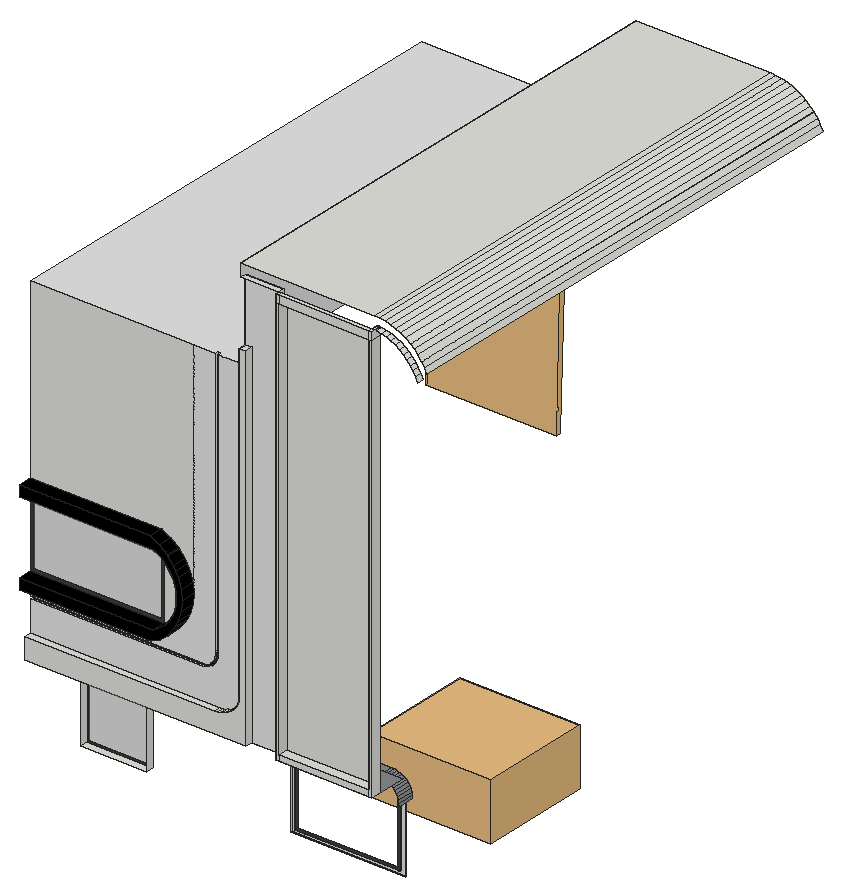
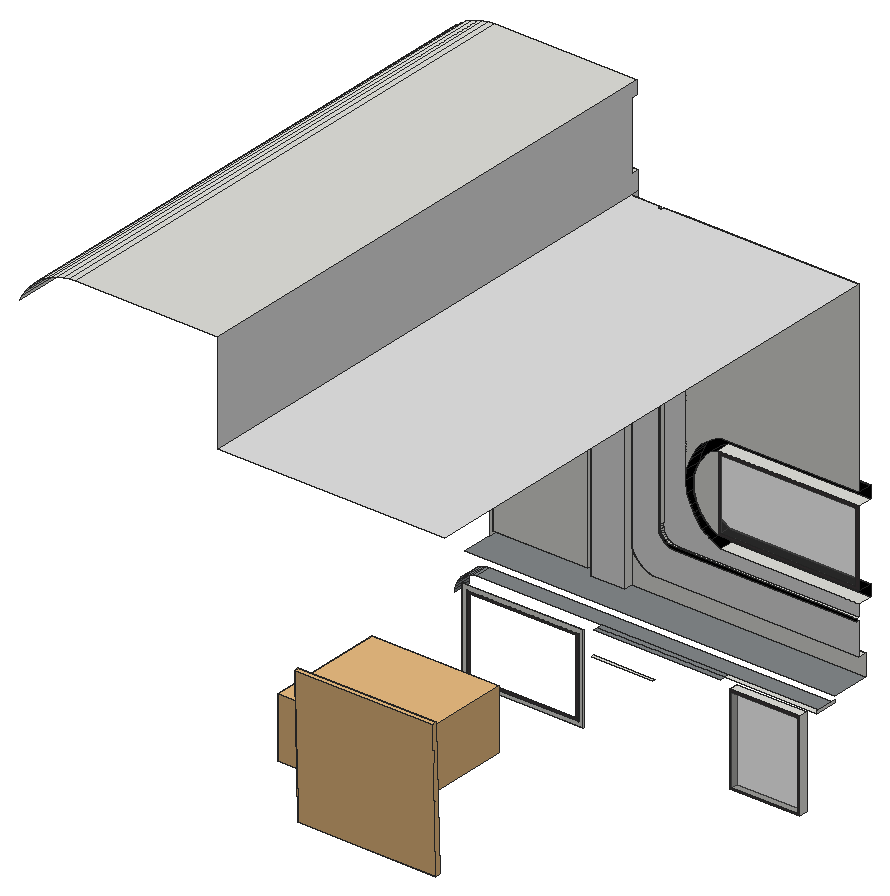
# SketchUp Ruby script. Lengths in inches.
U = 1.inch
M = Sketchup.active_model
def pt(a) = Geom::Point3d.new(a.map { |v| v * U })
def face(e, loops, mat)
  f = e.add_face(loops[0].map { |a| pt(a) })
  loops[1..].each { |l| e.add_face(l.map { |a| pt(a) }).erase! }
  f.material = f.back_material = mat if mat
  f
end
# faces: each face lists its corners as indices into pts; further lists are holes
def faces(e, pts, list, mat = nil) = list.each { |f| face(e, (f[0].is_a?(Array) ? f : [f]).map { |l| l.map { |i| pts[i] } }, mat) }
# xy, xz, yz: faces in a plane at the given z, y or x. An outline is a flat list of corners, or four numbers for a rectangle; further outlines are holes
def ring(l) = l.size == 4 ? [[l[0], l[1]], [l[2], l[1]], [l[2], l[3]], [l[0], l[3]]] : l.each_slice(2).to_a
def flat(e, list, mat, &to3) = list.each { |f| face(e, (f[0].is_a?(Array) ? f : [f]).map { |l| ring(l).map { |u, v| to3.(u, v) } }, mat) }
def xy(e, z, list, mat = nil) = flat(e, list, mat) { |x, y| [x, y, z] }
def xz(e, y, list, mat = nil) = flat(e, list, mat) { |x, z| [x, y, z] }
def yz(e, x, list, mat = nil) = flat(e, list, mat) { |y, z| [x, y, z] }
def lines(e, pts, list) = list.each { |a, b| e.add_line(pt(pts[a]), pt(pts[b])) }
# prism: a flat outline (further loops are holes) pulled along v
def prism(e, loops, v, mat = nil)
  f = face(e, loops, mat); d = Geom::Vector3d.new(v.map { |x| x * U })
  f.pushpull(f.normal.samedirection?(d) ? d.length : -d.length)
end
def box(e, o, s, mat = nil) = prism(e, [[o, [o[0] + s[0], o[1], o[2]], [o[0] + s[0], o[1] + s[1], o[2]], [o[0], o[1] + s[1], o[2]]]], [0, 0, s[2]], mat)
def at(x, y, z, deg = 0) = Geom::Transformation.translation(pt([x, y, z])) * Geom::Transformation.rotation(ORIGIN, Z_AXIS, deg.degrees)
def axes(o, x, y, z) = Geom::Transformation.new([*x, 0, *y, 0, *z, 0, *pt(o).to_a, 1])
def part(name) = M.definitions.add(name)
# library, detail: a bought-in or finely detailed component or shape, given as its bounding box
def library(name, o, s) = part(name).tap { |d| box(d.entities, o, s) }
def detail(e, o, s) = box(e.add_group.entities, o, s)
def put(e, d, t, mat = nil) = e.add_instance(d, t).tap { |i| i.material = mat if mat }
def group(e, t, mat = nil) = e.add_group.tap { |g| g.transformation = t; g.material = mat if mat }.entities
root = M.entities
M.materials.add("Black").color = [0, 0, 0]
M.materials.add("[Asphalt New]").color = [67, 60, 62]
M.materials.add("[Blacktop Old 01]").color = [132, 136, 139]
M.materials.add("[Polished Concrete Old]").color = [229, 229, 229]
M.materials.add("[Translucent Glass Gray]").color = [128, 128, 128]
M.materials["[Translucent Glass Gray]"].alpha = 0.5
c1 = library("koltuk",[-3.9375,-6.3,1.57],[103.3,102.81,49.85])
c2 = library("Trapezio",[0,0,0],[32.36,32.36,1.13])
xy(root,6.055,[[223.8,243.402,278.487,243.652]])
xy(root,7.284,[[123.071,243.402,154.634,247.34]])
xy(root,7.513,[[225.837,243.402,276.275,243.652]])
xy(root,40.089,[[187.79,247.965,215.602,249.09]])
xy(root,43.451,[[225.837,243.402,276.275,243.652]])
xy(root,45.43,[[223.8,243.402,278.487,243.652]])
xy(root,47.659,[[123.071,243.402,154.634,247.34]])
xy(root,50.25,[[116.615,243.402,158.149,245.465]])
xy(root,50.25,[[116.615,235.715,272.073,243.402],[158.149,243.402,215.602,245.465],[158.149,245.465,215.602,247.965]],"[Blacktop Old 01]")
xy(root,53.067,[[237.513,217.152,237.513,221.902,222.138,221.902,222.138,218.215,116.615,218.215,116.615,235.715,283.369,235.715,283.369,217.152]],"[Blacktop Old 01]")
xy(root,55.807,[[238.838,217.152,282.032,221.902]])
xy(root,62.745,[[116.615,218.215,207.152,221.902]])
xy(root,77.42,[[116.615,221.902,198.194,223.277]])
xy(root,78.866,[[116.615,221.902,198.793,223.277],[202.55,221.902,202.747,223.277]])
xy(root,84.302,[[116.615,215.402,179.295,221.902]])
xy(root,89.547,[[116.615,215.402,180.338,221.902]],"Black")
xy(root,123.86,[[116.615,215.402,180.338,221.902]])
xy(root,129.353,[[116.615,215.402,179.295,221.902]],"Black")
xy(root,213.5625,[[116.615,221.902,204.832,221.902,204.832,223.277,206.052,223.277,206.052,221.902,219.138,221.902,219.138,455.527,116.615,455.527]],"[Polished Concrete Old]")
xy(root,222.3125,[[219.138,218.215,222.138,221.902]])
xy(root,248.6875,[[238.838,217.152,282.032,221.902]])
xy(root,252.674,[[237.513,217.152,238.838,218.965],[238.838,217.152,282.032,218.965],[219.138,218.965,237.513,221.902],[282.032,218.965,283.369,221.902]])
xy(root,258.75,[[219.138,218.965,283.369,455.527]])
xz(root,215.402,[[116.615,84.302,179.295,84.302,183.559,86.518,187.303,89.532,187.316,89.547,190.379,93.224,191.302,94.93,192.666,97.451,194.076,102.045,194.552,106.827,194.076,111.61,192.666,116.204,191.302,118.725,190.379,120.431,187.522,123.86,187.303,124.123,183.559,127.137,179.295,129.353,116.615,129.353,116.615,123.86,180.338,123.86,183.429,122.056,186.124,119.703,188.327,116.884,189.96,113.7,190.964,110.266,191.302,106.704,190.964,103.142,189.96,99.707,188.327,96.524,186.124,93.704,183.429,91.351,180.338,89.547,116.615,89.547]],"Black")
xz(root,217.152,[[237.513,53.067,238.838,248.6875],[238.838,53.067,282.032,55.807],[282.032,53.067,283.369,248.6875],[237.513,248.6875,238.838,252.674],[238.838,248.6875,282.032,252.674],
  [282.032,248.6875,283.369,248.6875,283.369,252.57,282.032,252.674]])
xz(root,218.215,[[116.615,53.067,222.138,53.067,222.138,222.3125,219.138,222.3125,219.138,71.272,218.647,70.061,218.033,68.907,217.304,67.822,216.467,66.818,215.531,65.906,214.507,65.094,213.404,64.392,212.235,63.808,211.013,63.346,209.749,63.013,208.457,62.812,207.152,62.745,116.615,62.745]])
xz(root,221.902,[[238.838,55.807,282.032,248.6875],[202.55,78.866,202.747,78.866,202.765,78.88],[204.825,81.044,204.832,81.056,204.832,81.148],[180.338,89.547,183.429,91.351,186.124,93.704,188.327,96.524,189.96,99.707,190.964,103.142,191.302,106.704,190.964,110.266,189.96,113.7,188.327,116.884,186.124,119.703,183.429,122.056,180.338,123.86],[194.552,106.827,194.552,213.5625,116.615,213.5625,116.615,129.353,179.295,129.353,183.559,127.137,187.303,124.123,187.522,123.86,190.379,120.431,191.302,118.725,192.666,116.204,194.076,111.61],
  [283.369,252.57,283.369,252.674,282.032,252.674]])
xz(root,221.902,[[[116.615,89.547,180.338,123.86],[117.84,90.773,179.113,122.635]]],"[Asphalt New]")
xz(root,221.902,[[222.138,53.067,237.513,53.067,237.513,252.674,219.138,252.674,219.138,222.3125,222.138,222.3125],[116.615,62.745,207.152,62.745,208.457,62.812,209.749,63.013,211.013,63.346,212.235,63.808,213.404,64.392,214.507,65.094,215.531,65.906,216.467,66.818,217.304,67.822,218.033,68.907,218.647,70.061,219.138,71.272,219.138,213.5625,206.052,213.5625,206.052,84.566,205.9,83.607,205.633,82.675,205.253,81.782,204.832,81.056,204.825,81.044,204.766,80.942,204.18,80.169,203.504,79.474,202.765,78.88,202.747,78.866,201.922,78.356,201.04,77.951,200.116,77.658,199.162,77.48,198.194,77.42,116.615,77.42],[116.615,78.866,198.793,78.866,199.68,78.93,200.548,79.123,201.379,79.438,202.155,79.871,202.861,80.411,203.482,81.048,204.003,81.768,204.416,82.556,204.709,83.395,204.832,84.028,204.879,84.267,204.92,85.155,204.832,86.04,204.832,213.5625,194.552,213.5625,194.552,106.827,194.076,102.045,192.666,97.451,191.302,94.93,190.379,93.224,187.316,89.547,187.303,89.532,183.559,86.518,179.295,84.302,116.615,84.302]],"[Polished Concrete Old]")
xz(root,221.902,[[117.84,90.773,179.113,122.635]],"[Translucent Glass Gray]")
xz(root,223.277,[[116.615,77.42,198.194,77.42,199.162,77.48,200.116,77.658,201.04,77.951,201.922,78.356,202.747,78.866,202.55,78.866,202.765,78.88,203.504,79.474,204.18,80.169,204.766,80.942,204.825,81.044,204.832,81.148,204.832,81.056,205.253,81.782,205.633,82.675,205.9,83.607,206.052,84.566,206.052,213.5625,204.832,213.5625,204.832,86.04,204.92,85.155,204.879,84.267,204.832,84.028,204.709,83.395,204.416,82.556,204.003,81.768,203.482,81.048,202.861,80.411,202.155,79.871,201.379,79.438,200.548,79.123,199.68,78.93,198.793,78.866,116.615,78.866]],"Black")
xz(root,243.402,[[225.837,7.513,276.275,7.513,276.275,43.451,275.012,43.451,275.012,8.776,225.837,8.776],[225.837,8.776,227.1,8.776,227.1,42.1875,275.012,42.1875,275.012,43.451,225.837,43.451]],"[Asphalt New]")
xz(root,243.652,[[[223.8,6.055,278.487,45.43],[225.837,7.513,276.275,43.451]]])
xz(root,247.34,[[[123.071,7.284,154.634,47.659],[123.831,8.044,153.874,46.899]]],"[Asphalt New]")
xz(root,247.34,[[123.831,8.044,153.874,46.899]],"[Translucent Glass Gray]")
yz(root,116.615,[[235.715,50.25,245.465,51.308]])
yz(root,123.071,[[243.402,7.284,247.34,47.659]])
yz(root,154.634,[[243.402,7.284,247.34,47.659]])
yz(root,204.832,[[221.902,81.056,223.277,81.148],[221.902,86.04,223.277,213.5625]])
yz(root,206.052,[[221.902,84.566,223.277,213.5625]])
yz(root,219.138,[[218.215,71.272,221.902,213.5625],[218.215,213.5625,218.215,222.3125,221.902,222.3125,221.902,252.674,218.965,252.674,218.965,258.75,455.527,258.75,455.527,213.5625]],"[Polished Concrete Old]")
yz(root,222.138,[[218.215,53.067,221.902,222.3125]])
yz(root,223.8,[[243.402,6.055,243.652,45.43]])
yz(root,225.837,[[243.402,7.513,243.652,43.451]])
yz(root,237.513,[[217.152,53.067,221.902,248.6875],[217.152,248.6875,221.902,252.674]])
yz(root,238.838,[[217.152,55.807,221.902,248.6875]])
yz(root,276.275,[[243.402,7.513,243.652,43.451]])
yz(root,278.487,[[243.402,6.055,243.652,45.43]])
yz(root,282.032,[[217.152,55.807,221.902,248.6875]])
yz(root,283.369,[[217.152,53.067,221.902,248.6875],[217.152,248.6875,221.902,252.57],[218.965,252.57,221.902,252.674]])
p = [[281.715,243.402,41.795],[281.798,243.402,40.525],[281.798,235.715,40.525],[281.715,235.715,41.795],[281.467,243.402,43.042],[281.467,235.715,43.042],
  [281.058,243.402,44.247],[281.058,235.715,44.247],[280.495,243.402,45.388],[280.495,235.715,45.388],[279.789,243.402,46.445],[279.789,235.715,46.445],
  [278.95,243.402,47.402],[278.95,235.715,47.402],[277.993,243.402,48.24],[277.993,235.715,48.24],[276.936,243.402,48.947],[276.936,235.715,48.947],
  [275.795,243.402,49.51],[275.795,235.715,49.51],[274.59,243.402,49.919],[274.59,235.715,49.919],[273.343,243.402,50.167],[273.343,235.715,50.167],
  [272.073,243.402,50.25],[272.073,235.715,50.25],[208.457,221.902,62.812],[207.152,221.902,62.745],[207.152,218.215,62.745],[208.457,218.215,62.812],
  [209.749,221.902,63.013],[209.749,218.215,63.013],[211.013,221.902,63.346],[211.013,218.215,63.346],[212.235,221.902,63.808],[212.235,218.215,63.808],
  [213.404,221.902,64.392],[213.404,218.215,64.392],[214.507,221.902,65.094],[214.507,218.215,65.094],[215.531,221.902,65.906],[215.531,218.215,65.906],
  [216.467,221.902,66.818],[216.467,218.215,66.818],[217.304,221.902,67.822],[217.304,218.215,67.822],[218.033,221.902,68.907],[218.033,218.215,68.907],
  [218.647,221.902,70.061],[218.647,218.215,70.061],[219.138,221.902,71.272],[219.138,218.215,71.272],[198.194,221.902,77.42],[199.162,221.902,77.48],
  [199.162,223.277,77.48],[198.194,223.277,77.42],[200.116,221.902,77.658],[200.116,223.277,77.658],[201.04,221.902,77.951],[201.04,223.277,77.951],
  [201.922,221.902,78.356],[201.922,223.277,78.356],[202.747,221.902,78.866],[202.747,223.277,78.866],[199.68,221.902,78.93],[198.793,221.902,78.866],
  [198.793,223.277,78.866],[199.68,223.277,78.93],[200.548,221.902,79.123],[200.548,223.277,79.123],[202.55,221.902,78.866],[202.765,221.902,78.88],
  [202.765,223.277,78.88],[202.55,223.277,78.866],[203.504,221.902,79.474],[203.504,223.277,79.474],[201.379,221.902,79.438],[201.379,223.277,79.438],
  [202.155,221.902,79.871],[202.155,223.277,79.871],[204.18,221.902,80.169],[204.18,223.277,80.169],[202.861,221.902,80.411],[202.861,223.277,80.411],
  [204.766,221.902,80.942],[204.766,223.277,80.942],[203.482,221.902,81.048],[203.482,223.277,81.048],[204.825,221.902,81.044],[204.825,223.277,81.044],
  [204.003,221.902,81.768],[204.003,223.277,81.768],[204.832,221.902,81.148],[204.832,223.277,81.148],[204.832,221.902,81.056],[205.253,221.902,81.782],
  [205.253,223.277,81.782],[204.832,223.277,81.056],[204.416,221.902,82.556],[204.416,223.277,82.556],[205.633,221.902,82.675],[205.633,223.277,82.675],
  [204.709,221.902,83.395],[204.709,223.277,83.395],[205.9,221.902,83.607],[205.9,223.277,83.607],[204.832,221.902,84.028],[204.832,223.277,84.028],
  [206.052,221.902,84.566],[206.052,223.277,84.566],[204.879,221.902,84.267],[204.879,223.277,84.267],[179.295,221.902,84.302],[183.559,221.902,86.518],
  [183.559,215.402,86.518],[179.295,215.402,84.302],[204.92,221.902,85.155],[204.92,223.277,85.155],[204.832,221.902,86.04],[204.832,223.277,86.04],
  [187.303,221.902,89.532],[187.303,215.402,89.532],[183.429,221.902,91.351],[180.338,221.902,89.547],[180.338,215.402,89.547],[183.429,215.402,91.351],
  [187.316,221.902,89.547],[187.316,215.402,89.547],[190.379,221.902,93.224],[190.379,215.402,93.224],[186.124,221.902,93.704],[186.124,215.402,93.704],
  [191.302,221.902,94.93],[191.302,215.402,94.93],[188.327,221.902,96.524],[188.327,215.402,96.524],[192.666,221.902,97.451],[192.666,215.402,97.451],
  [189.96,221.902,99.707],[189.96,215.402,99.707],[194.076,221.902,102.045],[194.076,215.402,102.045],[190.964,221.902,103.142],[190.964,215.402,103.142],
  [194.552,221.902,106.827],[194.552,215.402,106.827],[191.302,221.902,106.704],[191.302,215.402,106.704],[190.964,221.902,110.266],[190.964,215.402,110.266],
  [194.076,221.902,111.61],[194.076,215.402,111.61],[189.96,221.902,113.7],[189.96,215.402,113.7],[192.666,221.902,116.204],[192.666,215.402,116.204],
  [188.327,221.902,116.884],[188.327,215.402,116.884],[191.302,221.902,118.725],[191.302,215.402,118.725],[186.124,221.902,119.703],[186.124,215.402,119.703],
  [190.379,221.902,120.431],[190.379,215.402,120.431],[183.429,221.902,122.056],[183.429,215.402,122.056],[187.522,221.902,123.86],[187.522,215.402,123.86],
  [180.338,221.902,123.86],[180.338,215.402,123.86],[187.303,221.902,124.123],[187.303,215.402,124.123],[183.559,221.902,127.137],[183.559,215.402,127.137],
  [179.295,221.902,129.353],[179.295,215.402,129.353],[302.995,221.902,239.289],[303.95,221.902,237.116],[303.95,218.965,237.116],[302.995,218.965,239.289],
  [301.832,221.902,241.358],[301.832,218.965,241.358],[300.472,221.902,243.304],[300.472,218.965,243.304],[307.165,455.527,244.707],[307.165,218.965,244.707],
  [308.325,218.965,242.342],[308.325,455.527,242.342],[298.927,221.902,245.106],[298.927,218.965,245.106],[305.781,455.527,246.948],[305.781,218.965,246.948],
  [297.214,221.902,246.749],[297.214,218.965,246.749],[295.348,221.902,248.216],[295.348,218.965,248.216],[304.1875,455.527,249.045],[304.1875,218.965,249.045],
  [293.348,221.902,249.494],[293.348,218.965,249.494],[303.95,455.527,249.302],[303.95,218.965,249.302],[302.398,455.527,250.978],[302.398,218.965,250.978],
  [291.232,221.902,250.569],[291.232,218.965,250.569],[289.02,221.902,251.432],[289.02,218.965,251.432],[300.492,455.527,252.674],[300.492,218.965,252.674],
  [286.735,221.902,252.074],[286.735,218.965,252.074],[284.398,221.902,252.49],[284.398,218.965,252.49],[283.369,221.902,252.57],[283.369,218.965,252.57],
  [282.032,221.902,252.674],[282.032,218.965,252.674],[282.032,217.152,252.674],[283.369,217.152,252.57],[298.302,455.527,254.281],[298.302,218.965,254.281],
  [300.43,218.965,252.729],[300.43,455.527,252.729],[296.034,455.527,255.619],[296.034,218.965,255.619],[293.646,455.527,256.732],[293.646,218.965,256.732],
  [291.163,455.527,257.609],[291.163,218.965,257.609],[288.606,455.527,258.241],[288.606,218.965,258.241],[286,455.527,258.622],[286,218.965,258.622],
  [283.369,455.527,258.75],[283.369,218.965,258.75]]
faces(root,p,[[0,1,2,3],[4,0,3,5],[6,4,5,7],[8,6,7,9],[10,8,9,11],[12,10,11,13],[14,12,13,15],[16,14,15,17],
  [18,16,17,19],[20,18,19,21],[22,20,21,23],[24,22,23,25]],"[Blacktop Old 01]")
faces(root,p,[[26,27,28,29],[30,26,29,31],[32,30,31,33],[34,32,33,35],[36,34,35,37],[38,36,37,39],[40,38,39,41],[42,40,41,43],
  [44,42,43,45],[46,44,45,47],[48,46,47,49],[50,48,49,51],[52,53,54,55],[53,56,57,54],[56,58,59,57],[58,60,61,59],
  [60,62,63,61],[64,65,66,67],[68,64,67,69],[70,71,72,73],[71,74,75,72],[76,68,69,77],[78,76,77,79],[74,80,81,75],
  [82,78,79,83],[80,84,85,81],[86,82,83,87],[84,88,89,85],[90,86,87,91],[88,92,93,89],[94,95,96,97],[98,90,91,99],
  [95,100,101,96],[102,98,99,103],[100,104,105,101],[106,102,103,107],[104,108,109,105],[110,106,107,111],[116,110,111,117],[118,116,117,119],
  [176,177,178,179],[180,176,179,181],[182,180,181,183],[184,185,186,187],[188,182,183,189],[190,191,185,184],[192,188,189,193],[194,192,193,195],
  [196,197,191,190],[198,194,195,199],[200,201,197,196],[202,203,201,200],[204,198,199,205],[206,204,205,207],[208,209,203,202],[210,206,207,211],
  [212,210,211,213],[214,212,213,215],[214,216,217,218,219,215],[220,221,222,223],[223,222,209,208],[224,225,221,220],[226,227,225,224],[228,229,227,226],
  [230,231,229,228],[232,233,231,230],[234,235,233,232]])
faces(root,p,[[112,113,114,115],[113,120,121,114],[122,123,124,125],[120,126,127,121],[126,128,129,127],[130,122,125,131],[128,132,133,129],[134,130,131,135],
  [132,136,137,133],[138,134,135,139],[136,140,141,137],[142,138,139,143],[140,144,145,141],[146,142,143,147],[148,146,147,149],[144,150,151,145],
  [152,148,149,153],[150,154,155,151],[156,152,153,157],[154,158,159,155],[160,156,157,161],[158,162,163,159],[164,160,161,165],[162,166,167,163],
  [168,164,165,169],[166,170,171,167],[170,172,173,171],[172,174,175,173]],"Black")
put(root,c1,axes([236.41,330.92,7.48],[0,-0.51724,0],[0.55845,0,0],[0,0,0.54735]))
put(root,c2,axes([186.4375,451.03,71.96],[0,0.06735,1.92436],[-1.92554,0,0],[0,-1.92436,0.06735]))
